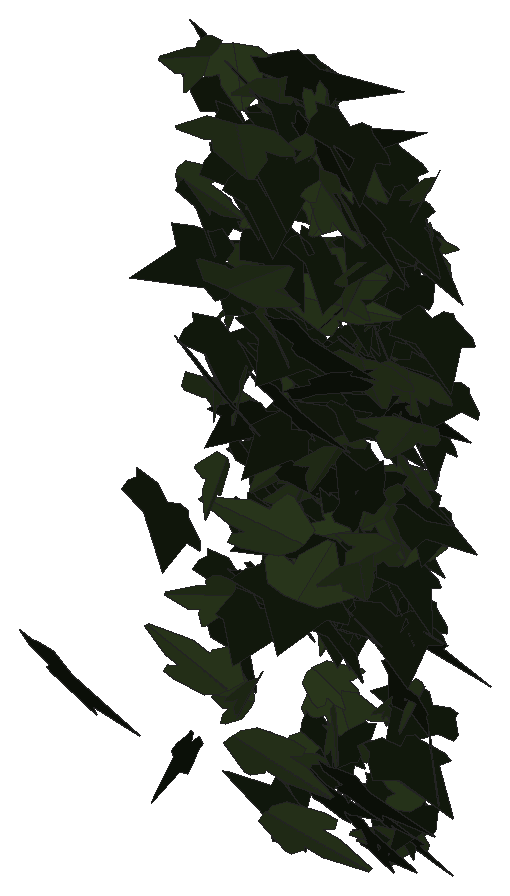
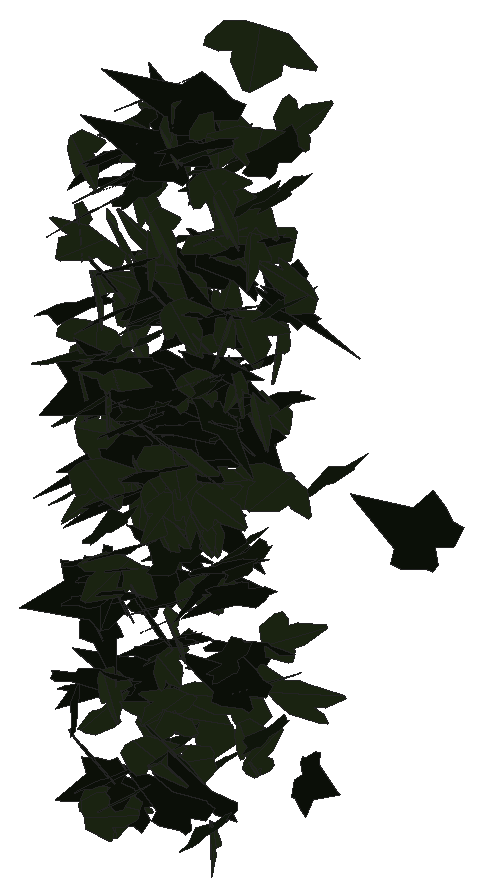
# SketchUp Ruby script. Lengths in millimetres.
U = 1.mm
M = Sketchup.active_model
def pt(a) = Geom::Point3d.new(a.map { |v| v * U })
def face(e, loops, mat)
  f = e.add_face(loops[0].map { |a| pt(a) })
  loops[1..].each { |l| e.add_face(l.map { |a| pt(a) }).erase! }
  f.material = f.back_material = mat if mat
  f
end
# faces: each face lists its corners as indices into pts; further lists are holes
def faces(e, pts, list, mat = nil) = list.each { |f| face(e, (f[0].is_a?(Array) ? f : [f]).map { |l| l.map { |i| pts[i] } }, mat) }
# xy, xz, yz: faces in a plane at the given z, y or x. An outline is a flat list of corners, or four numbers for a rectangle; further outlines are holes
def ring(l) = l.size == 4 ? [[l[0], l[1]], [l[2], l[1]], [l[2], l[3]], [l[0], l[3]]] : l.each_slice(2).to_a
def flat(e, list, mat, &to3) = list.each { |f| face(e, (f[0].is_a?(Array) ? f : [f]).map { |l| ring(l).map { |u, v| to3.(u, v) } }, mat) }
def xy(e, z, list, mat = nil) = flat(e, list, mat) { |x, y| [x, y, z] }
def xz(e, y, list, mat = nil) = flat(e, list, mat) { |x, z| [x, y, z] }
def yz(e, x, list, mat = nil) = flat(e, list, mat) { |y, z| [x, y, z] }
def lines(e, pts, list) = list.each { |a, b| e.add_line(pt(pts[a]), pt(pts[b])) }
# prism: a flat outline (further loops are holes) pulled along v
def prism(e, loops, v, mat = nil)
  f = face(e, loops, mat); d = Geom::Vector3d.new(v.map { |x| x * U })
  f.pushpull(f.normal.samedirection?(d) ? d.length : -d.length)
end
def box(e, o, s, mat = nil) = prism(e, [[o, [o[0] + s[0], o[1], o[2]], [o[0] + s[0], o[1] + s[1], o[2]], [o[0], o[1] + s[1], o[2]]]], [0, 0, s[2]], mat)
def at(x, y, z, deg = 0) = Geom::Transformation.translation(pt([x, y, z])) * Geom::Transformation.rotation(ORIGIN, Z_AXIS, deg.degrees)
def axes(o, x, y, z) = Geom::Transformation.new([*x, 0, *y, 0, *z, 0, *pt(o).to_a, 1])
def part(name) = M.definitions.add(name)
# library, detail: a bought-in or finely detailed component or shape, given as its bounding box
def library(name, o, s) = part(name).tap { |d| box(d.entities, o, s) }
def detail(e, o, s) = box(e.add_group.entities, o, s)
def put(e, d, t, mat = nil) = e.add_instance(d, t).tap { |i| i.material = mat if mat }
def group(e, t, mat = nil) = e.add_group.tap { |g| g.transformation = t; g.material = mat if mat }.entities
root = M.entities
M.materials.add("efeu1").color = [18, 25, 13]
M.materials.add("efeu2").color = [43, 57, 29]
c1 = part("ivyleaf_9")
p = [[39.1,54.8,31.7],[34.5,51.8,30.2],[-5.3,25.2,17.3],[-17.9,28.3,20.9],[-21.6,21.7,17],[-20.2,4.3,5.3],
  [-22.9,-0.3,2.5],[-17.1,-4,-0.6],[-2,-2.1,-1.2],[-0.7,-15.4,-10.1],[16.6,-22.3,-16.7],[21.1,-15.1,-12.5],
  [32.7,-10.7,-11],[46.1,-1.8,-6.6],[30.8,11.2,3.8]]
faces(c1.entities,p,[[0,1,2,3,4,5,6,7,8,9,10,11,12,13,14]],"efeu1")
c2 = part("ivyleaf_10")
p = [[0,12.8,-0.8],[-1.5,51.3,-10.9],[-4.9,51,-11.6],[-13.6,26.5,-7.3],[-13.2,15.9,-4.6],[-21.1,19.3,-7.2],
  [-29.5,16.3,-8.3],[-29.2,8.3,-6.2],[-19.7,-9.8,0.5],[-7.6,-13,4],[1,-12.2,5.8],[-0.4,51.1,-11.1],
  [-1.5,51.1,-10.9],[1,-12.4,5.9],[16.9,-12.4,3.5],[35.1,9.1,-5.1],[35,12.9,-6.1],[20.5,16.4,-4.9],
  [15.8,15,-3.8],[15.3,27.6,-7.1],[12.8,31.3,-7.8]]
faces(c2.entities,p,[[0,1,2,3,4,5,6,7,8,9,10],[11,12,0,13,14,15,16,17,18,19,20]],"efeu2")
put(root,c1,axes([2602.7,851.9,2372.3],[-0.21936,-0.87871,0.39416],[0.01495,-0.39782,-0.88456],[1.83284,-0.10192,0.05439]))
put(root,c1,axes([2606,888.9,1878.8],[-0.45994,-0.83129,0.24224],[0.0835,-0.26293,-0.85853],[1.64581,-0.21897,0.11125]))
put(root,c1,axes([2597.8,883.8,1811],[0.40132,-0.8507,0.15451],[0.01269,-0.15743,-0.8759],[1.64549,0.20869,-0.03093]))
put(root,c2,axes([2606.7,848.6,2133.5],[-1.77967,0.18399,-0.36635],[0.68472,-0.06912,-0.95302],[-0.37405,-1.00191,-0.00152]))
put(root,c2,axes([2620.8,872.2,2243.8],[0.1641,-0.95502,-0.15053],[0.02834,0.15242,-0.95849],[1.83982,0.08284,0.02819]))
put(root,c1,axes([2618.1,790.3,1709],[-0.44208,0.13684,-0.98546],[1.08797,-0.80989,-0.24721],[-1.54976,-0.60759,0.10757]))
put(root,c2,axes([2629.9,801.5,2581.4],[-0.29414,-0.27137,-1.10559],[-0.80082,-1.0231,0.30995],[-2.01318,0.44662,0.03824]))
put(root,c2,axes([2587.1,834.3,2392.7],[-0.07253,0.03539,-1.04948],[1.52236,-0.6794,-0.05196],[-1.29477,-0.8008,-0.0023]))
put(root,c2,axes([2650.2,790.4,1807.9],[1.21959,0.24218,0.89079],[-1.66786,-0.18121,0.67969],[0.55217,-1.08227,0.08553]))
put(root,c2,axes([2641.4,816.1,1895.3],[-0.17895,-0.14003,-1.00925],[-1.12514,-0.818,0.16857],[-1.57943,0.59859,-0.00574]))
put(root,c1,axes([2602.5,840.2,2524.3],[0.83467,-0.89447,-0.20918],[-0.04957,0.2196,-0.99361],[1.74759,0.43344,0.07172]))
put(root,c1,axes([2662.7,790.7,2338.8],[-1.96485,0.28691,0.1811],[-0.33956,0.0343,-1.07142],[-0.54924,-1.04759,0.01452]))
put(root,c1,axes([2615.8,893,2042],[0.65257,-0.84782,0.1484],[0.10051,-0.13872,-0.91452],[1.63502,0.34691,-0.00301]))
put(root,c2,axes([2641.4,857.5,2446],[0.06645,-0.87731,-0.49535],[0.1631,0.49643,-0.87319],[1.91051,-0.01187,0.09177]))
put(root,c1,axes([2613.3,848.2,2566.1],[0.38578,-0.74441,0.64559],[0.59711,-0.57604,-0.76273],[1.77773,0.35503,0.11609]))
put(root,c2,axes([2642.1,853.7,1748],[-0.18778,0.52923,0.88057],[0.34196,-0.8621,0.53826],[1.92516,0.20476,-0.00972]))
put(root,c2,axes([2649.5,882.2,2285.5],[0.87392,-0.77091,-0.40072],[-0.12709,0.42059,-0.88565],[1.64868,0.44106,0.14414]))
put(root,c2,axes([2645.8,875.2,2272.1],[-0.96305,0.80714,0.03517],[-0.01761,0.03571,-0.95257],[-1.5375,-0.50598,-0.01112]))
put(root,c1,axes([2653.1,906.9,2031.1],[-0.85704,-0.76995,0.24056],[-0.14302,-0.23427,-0.89048],[1.52855,-0.45362,0.05156]))
put(root,c1,axes([2646.3,825.7,2223.9],[-0.62993,-0.91874,-0.13351],[0.05549,0.13138,-0.9764],[1.76605,-0.33184,-0.01694]))
put(root,c2,axes([2659.9,848.3,1776],[0.00096,-0.95236,0.04986],[0.00034,-0.04986,-0.95236],[1.815,0.00052,0.00015]))
put(root,c2,axes([2667.4,845.8,2326.4],[-1.12713,-0.8143,0.204],[-0.15951,-0.19105,-1.00594],[1.58969,-0.59653,0.0437]))
put(root,c1,axes([2624.7,891.2,1862.4],[0.54599,-0.24385,0.81417],[1.25459,-0.47854,-0.37561],[1.02098,0.71844,0.02616]))
put(root,c1,axes([2646.8,713.2,2059],[-0.25549,-1.02864,0.62561],[-0.07671,-0.62529,-1.03677],[2.29006,-0.13571,0.03507]))
put(root,c1,axes([2641.6,871.1,1986.9],[0.34993,-0.51268,-0.7806],[0.08361,0.79945,-0.51472],[1.77544,0.0634,0.17809]))
put(root,c2,axes([2659,879.3,2336.6],[0.33743,-0.68183,-0.69468],[0.3058,0.71692,-0.66265],[1.82712,0.00593,0.2392]))
put(root,c1,axes([2680.8,894.3,2292.9],[-1.79147,-0.1632,0.03486],[-0.07173,0.01332,-0.95514],[0.30941,-0.94185,-0.01955]))
put(root,c2,axes([2652.5,829.2,2576.8],[1.51932,0.76395,0.04593],[0.06434,0.03111,-1.10495],[-1.45516,0.79901,-0.0009]))
put(root,c1,axes([2619,549,1914.7],[0.94474,-0.72214,0.98745],[1.06901,-0.81214,-0.8763],[2.06833,0.7496,0.00188]))
put(root,c1,axes([2683.1,877,2215.3],[-0.61302,0.88597,-0.01251],[0.01307,-0.01081,-0.9427],[-1.6863,-0.32216,-0.00276]))
put(root,c1,axes([2655.4,843.9,2435.6],[-0.35308,-1.00084,-0.11203],[0.0424,0.10981,-1.01789],[1.91623,-0.18684,0.00188]))
put(root,c1,axes([2650.6,852.8,2279],[0.34682,-0.92077,-0.42788],[-0.10101,0.42548,-0.93822],[1.92974,0.18776,0.02779]))
put(root,c1,axes([2648.3,883.3,1894.6],[0.94182,-0.7498,0.06909],[0.0776,-0.05587,-0.89837],[1.43095,0.49653,0.00325]))
put(root,c1,axes([2656.4,839,2487.8],[0.17531,-0.969,0.27289],[0.08006,-0.27008,-0.97324],[1.91426,0.10004,0.01571]))
put(root,c2,axes([2678.5,869.3,2488],[0.44902,-0.97411,0.15207],[0.06468,-0.14824,-1.00227],[1.87527,0.23836,-0.00184]))
put(root,c1,axes([2680.4,834.6,1882.8],[-1.20928,-0.64803,-0.07539],[0.10298,0.05252,-0.90756],[1.23736,-0.63769,0.00186]))
put(root,c2,axes([2682.5,880.9,1649.4],[0.44059,-0.74472,-0.50283],[0.01518,0.52094,-0.76786],[1.71011,0.18724,0.13637]))
put(root,c2,axes([2670.6,816.1,2182],[0.70923,-0.63127,0.66398],[0.68561,-0.55811,-0.73279],[1.60321,0.51793,0.01964]))
put(root,c2,axes([2681.4,822.4,2472.4],[-1.96824,0.26821,-0.24851],[0.45899,-0.06,-1.06839],[-0.52306,-1.06192,-0.0024]))
put(root,c1,axes([2673.2,906.2,1661.4],[0.07009,-0.86836,0.3748],[-0.0412,-0.37576,-0.86845],[1.79955,0.02522,-0.03448]))
put(root,c1,axes([2708.5,811.3,2153.3],[0.26368,0.62848,-0.82882],[-0.47805,-0.79118,-0.64192],[-1.92103,0.28315,0.04598]))
put(root,c2,axes([2698.6,865.8,2512.7],[-0.7251,-0.88498,0.32547],[-0.01409,-0.34822,-0.95549],[1.79453,-0.36032,0.12401]))
put(root,c1,axes([2676.6,825.7,2014.3],[0.85335,-0.85765,-0.3751],[-0.31251,0.3374,-0.96773],[1.75394,0.47739,0.01007]))
put(root,c1,axes([2690.4,868.7,1986.1],[0.63778,-0.48439,-0.83189],[-0.76032,0.73144,-0.58683],[1.66688,0.51897,0.05062]))
put(root,c1,axes([2680.7,874.8,2256.2],[0.32728,-0.92549,0.15648],[0.03045,-0.15617,-0.94125],[1.78614,0.17224,-0.01263]))
put(root,c2,axes([2711.2,854.1,2075.8],[-0.36736,-0.69607,0.67241],[-0.26741,-0.65823,-0.72173],[1.82242,-0.2369,0.02964]))
put(root,c1,axes([2675.1,845.6,2196.2],[0.85438,-0.86585,0.1528],[0.15317,-0.13038,-0.97524],[1.66632,0.45593,0.0113]))
put(root,c2,axes([2711.2,838.5,2421.2],[1.3122,0.52505,-0.56863],[-0.85221,-0.35053,-0.86661],[-1.20145,0.82209,-0.00634]))
put(root,c1,axes([2709.9,900.4,2196.5],[-1.12055,-0.74701,0.11521],[-0.07552,-0.11529,-0.95031],[1.43654,-0.58876,0.03991]))
put(root,c1,axes([2705.1,874.1,2249],[-0.63639,-0.80058,0.39494],[-0.09437,-0.40443,-0.8618],[1.69635,-0.32284,0.10022]))
put(root,c1,axes([2700.3,827.6,2427.8],[-0.36829,-0.99153,0.12935],[0.03974,-0.13573,-1.00919],[1.90266,-0.18909,0.04612]))
put(root,c2,axes([2712.3,714.3,2237.3],[0.75529,-0.74713,-0.71349],[0.11803,0.78017,-0.78246],[1.96263,0.2406,0.32163]))
put(root,c2,axes([2716.1,824.3,2567.7],[-1.07398,-0.83663,-0.16183],[0.17456,0.13334,-1.00915],[1.61237,-0.5717,0.00146]))
put(root,c2,axes([2721.8,863.3,1959.1],[-0.8275,-0.6079,0.53089],[-0.03967,-0.59436,-0.69766],[1.53554,-0.34295,0.26807]))
put(root,c2,axes([2722.7,847.3,2043.2],[-0.2692,-0.89225,0.21418],[0.06119,-0.2214,-0.90107],[1.74529,-0.12986,0.06463]))
put(root,c2,axes([2720.2,863,2044.2],[-0.08012,-0.86376,0.32622],[0.16338,-0.32881,-0.85953],[1.74963,-0.00885,0.0952]))
put(root,c1,axes([2696.9,836.8,2511.4],[0.7449,-0.9047,-0.11968],[0.00858,0.13214,-0.98413],[1.7368,0.38737,0.05619]))
put(root,c2,axes([2727.2,891.9,2338.7],[-0.41673,-0.903,0.26053],[-0.09602,-0.25583,-0.9291],[1.7861,-0.22444,0.01084]))
put(root,c2,axes([2721.9,838.3,2309.6],[-1.54178,-0.6012,-0.27155],[0.40626,0.16801,-1.00879],[1.18797,-0.83771,-0.00744]))
put(root,c1,axes([2715.8,865.9,1675.8],[-1.2914,0.37308,0.5768],[0.89547,-0.33831,0.77232],[0.95258,0.82381,0.05594]))
put(root,c1,axes([2706.7,866.5,2327.1],[-0.17094,-0.77049,-0.6316],[0.25426,0.61912,-0.77427],[1.879,-0.15387,0.04731]))
put(root,c2,axes([2718.6,717.5,2126.7],[-0.02832,-0.76302,0.78628],[0.65781,-0.74947,-0.72075],[1.97875,0.23823,0.25086]))
put(root,c1,axes([2706,844.4,2301.6],[-0.46181,0.39278,0.92671],[0.71503,-0.84901,0.45822],[1.77714,0.44367,0.05645]))
put(root,c1,axes([2708.6,871.7,2564.9],[0.00716,-0.93278,-0.39109],[0.25402,0.38813,-0.92444],[1.90816,-0.04817,0.12453]))
put(root,c2,axes([2737.8,858.7,2074.8],[-0.29774,-1.00667,-0.02735],[0.01379,0.02656,-1.01875],[1.91656,-0.15658,0.00308]))
put(root,c2,axes([2735.3,893.7,1920.4],[0.64883,-0.83939,-0.00188],[0.00844,0.00383,-0.90596],[1.5975,0.3409,0.00555]))
put(root,c1,axes([2714.9,679.2,2280],[1.91372,-0.57363,-0.42942],[-0.70249,0.21958,-1.15762],[1.1689,1.07111,0.00734]))
put(root,c1,axes([2725.3,843.5,2533.8],[-0.56061,-0.83063,0.51097],[0.12107,-0.549,-0.85578],[1.85206,-0.21554,0.21061]))
put(root,c1,axes([2728.4,908.2,1932.4],[-0.35387,-0.84422,0.35375],[-0.10126,-0.3504,-0.86418],[1.73913,-0.19218,0.02166]))
put(root,c2,axes([2740.7,850.1,2219.7],[-0.52454,-0.83124,0.55958],[0.14083,-0.59566,-0.84839],[1.90188,-0.18515,0.21715]))
put(root,c1,axes([2748.8,801.8,2149.6],[-1.73822,0.19062,-0.36483],[0.67867,-0.07713,-0.93299],[-0.39134,-0.98046,0.00247]))
put(root,c2,axes([2765.7,769,2038.9],[0.76,0.52464,1.03967],[-1.26191,-0.80112,0.65893],[1.82204,-0.77368,0.0227]))
put(root,c2,axes([2738.4,902,1867.4],[-0.10446,-0.73977,0.53334],[0.31137,-0.53362,-0.72333],[1.70753,0.05205,0.16453]))
put(root,c1,axes([2717.8,813.2,2381.7],[-0.80055,-0.24656,-0.92627],[1.80363,0.04474,-0.44227],[0.27361,-1.01632,0.20525]))
put(root,c1,axes([2718.5,902.4,2012.7],[0.24235,-0.75514,0.53029],[0.43144,-0.49331,-0.75691],[1.70234,0.23253,0.11634]))
put(root,c1,axes([2745.7,829.3,2496.7],[-1.04861,-0.62266,0.728],[-0.35671,-0.75352,-0.78634],[1.78795,-0.51551,0.27008]))
put(root,c1,axes([2768.2,888.9,2160.2],[-1.62005,0.40612,0.03095],[-0.13797,-0.08051,-0.93741],[-0.7628,-0.84797,0.10382]))
put(root,c2,axes([2754.6,867.8,2125],[-1.59628,-0.38878,0.14588],[-0.2393,-0.07558,-0.92433],[0.7532,-0.84797,0.01551]))
put(root,c1,axes([2738.2,838.3,2476.9],[-0.36713,-0.03737,1.02446],[-0.1822,-1.03723,-0.05586],[1.94253,-0.10435,0.18838]))
put(root,c2,axes([2727.4,845.5,1715.9],[-0.15918,-0.11898,-0.91944],[1.17068,0.68359,-0.14442],[1.32016,-0.62053,0.0172]))
put(root,c1,axes([2773,842,2298.9],[-1.46345,0.3736,-0.61075],[-1.04256,0.27009,0.85489],[0.87737,0.94411,-0.00288]))
put(root,c1,axes([2775.5,805.3,2025.9],[0.43176,0.16561,-1.03235],[-1.4954,-0.66991,-0.28013],[-1.31279,0.81757,-0.02043]))
put(root,c1,axes([2762.3,793.9,1666.3],[-0.07811,-1.04362,-0.04959],[0.01653,-0.04997,1.04437],[-1.98839,0.04058,0.01063]))
put(root,c2,axes([2752.7,773.2,2270.5],[-1.58975,0.70766,0.13036],[0.17014,-0.09612,1.09466],[1.35887,0.83993,0.01545]))
put(root,c1,axes([2727.1,855.1,2015.3],[1.01737,-0.72192,-0.21192],[-0.05691,0.23937,-0.89086],[1.4308,0.52284,0.11525]))
put(root,c1,axes([2741.2,886.8,1891.1],[-0.46485,-0.86165,-0.14163],[0.054,0.13916,-0.89554],[1.66102,-0.24566,-0.01052]))
put(root,c1,axes([2736.1,883.2,2006.5],[0.4226,-0.8651,-0.19712],[-0.11894,0.18744,-0.89304],[1.68446,0.23027,-0.0136]))
put(root,c2,axes([2733.4,736.2,2355],[-1.6719,-0.55676,0.57833],[1.05221,0.20201,1.03426],[-1.10777,1.03216,0.10954]))
put(root,c1,axes([2754.6,820.9,1945.9],[-1.44548,-0.77644,-0.16308],[0.21474,0.11776,-1.08614],[1.49462,-0.76783,-0.00167]))
put(root,c2,axes([2759.5,879.9,2037.5],[1.33451,-0.53462,-0.30281],[-0.31051,0.28097,-0.87385],[1.12739,0.71022,0.11776]))
put(root,c2,axes([2749.6,873.3,2063.1],[-0.61232,-0.71471,-0.68752],[0.67291,0.59264,-0.78152],[1.7634,-0.47432,0.05949]))
put(root,c1,axes([2792.4,838.5,2171],[-1.75389,-0.20828,-0.4318],[-0.8026,-0.09281,0.94479],[-0.43395,1.01345,-0.00222]))
put(root,c1,axes([2749.1,890.3,1937.7],[-0.48016,-0.85266,0.19023],[0.07408,-0.20878,-0.88418],[1.66103,-0.23717,0.09442]))
put(root,c1,axes([2726.1,875,1655.5],[0.39822,-0.3432,0.85894],[1.08974,-0.64357,-0.39663],[1.38256,0.60612,0.06522]))
put(root,c2,axes([2745.4,869.7,1803.9],[0.53531,0.73337,0.51824],[0.38364,0.47764,-0.78532],[-1.66545,0.34575,-0.01433]))
put(root,c2,axes([2781.6,885.6,1727.4],[-0.88868,-0.4314,0.62761],[-0.87254,-0.42862,-0.63572],[1.15739,-0.65438,0.00264]))
put(root,c1,axes([2753.1,900.8,1886],[-0.47819,-0.88041,-0.04633],[0.02189,0.0449,-0.91556],[1.67778,-0.25152,-0.00126]))
put(root,c1,axes([2743,880.8,1879.2],[0.4374,-0.87455,0.01617],[0.00837,-0.01557,-0.90425],[1.66471,0.22987,0.0003]))
put(root,c2,axes([2770.3,875.4,2077],[-0.39273,-0.82514,0.38375],[-0.14479,-0.37647,-0.85041],[1.72587,-0.21935,0.01598]))
put(root,c1,axes([2791,840.8,2207.7],[-0.18523,0.05044,1.04927],[-1.90244,-0.32843,-0.07693],[0.61469,-1.00129,0.07809]))
put(root,c1,axes([2729.6,807.7,2176],[0.67307,-0.53428,0.84873],[0.97864,-0.67605,-0.63984],[1.63872,0.62318,0.03352]))
put(root,c1,axes([2769.2,790,2279.6],[-1.08532,-0.75318,0.37312],[-0.16461,-0.39592,-0.93138],[1.59121,-0.55468,0.15814]))
put(root,c2,axes([2772.3,870.8,2432.7],[0.24487,-0.99177,0.13567],[-0.00161,-0.1369,-0.99991],[1.90512,0.12736,-0.01828]))
put(root,c1,axes([2751.5,875.6,1734.7],[0.1275,-0.97796,0.37851],[0.02741,-0.37838,-0.98019],[1.99561,0.06768,-0.01072]))
put(root,c2,axes([2734.7,761,1761.1],[-1.14756,0.10314,-1.02967],[1.92973,-0.17936,-0.61172],[-0.39372,-1.17967,0.00298]))
put(root,c1,axes([2729.2,827.6,2574.8],[0.55015,-0.0248,1.07842],[2.02917,-0.16304,-0.28954],[0.31188,1.10452,-0.01853]))
put(root,c1,axes([2764.4,775.7,2516.5],[-0.61307,-1.05615,-0.06929],[0.03486,0.06685,-1.10418],[2.01409,-0.32264,-0.00198]))
put(root,c1,axes([2803.4,869.4,1914],[-0.88816,0.23696,-0.90256],[-1.59524,0.33707,0.52188],[0.78054,0.95852,0.0396]))
put(root,c2,axes([2769.6,857.2,2548.2],[0.63927,-0.83895,0.45568],[0.36289,-0.41437,-0.90346],[1.78041,0.38569,0.02053]))
put(root,c1,axes([2801.9,853.3,1746.5],[-1.02056,0.78745,0.25666],[-0.31157,0.19895,-0.95242],[-1.54517,-0.56021,0.02253]))
put(root,c1,axes([2768.9,878.4,2104.2],[-0.63357,-0.87532,-0.0189],[0.01434,0.01735,-0.93649],[1.66624,-0.33298,0.00088]))
put(root,c2,axes([2784.4,854.2,2011.3],[-0.26579,0.04739,0.94196],[-0.21679,-0.94611,0.03071],[1.78187,-0.10804,0.14424]))
put(root,c2,axes([2781.4,674.3,2594.8],[-2.21566,-0.48141,-0.08027],[0.13984,0.03237,-1.25978],[0.91829,-1.16649,-0.00183]))
put(root,c2,axes([2761.3,875.5,1777],[1.64432,0.29336,0.24652],[0.43303,0.09651,-0.91225],[-0.58681,0.89326,0.0176]))
put(root,c1,axes([2800.4,840.6,1987.9],[-2.00035,-0.0233,-0.03402],[0.06484,-0.00168,-1.0513],[0.04423,-1.0516,0.00243]))
put(root,c2,axes([2784,812.6,2553.7],[0.01539,0.67421,-0.8208],[0.07808,0.82001,0.67397],[2.02008,-0.03683,-0.01979]))
put(root,c1,axes([2740.3,809.6,2096],[0.69289,-0.12693,0.98829],[1.72891,-0.39001,-0.38473],[0.77912,0.97834,-0.02516]))
put(root,c1,axes([2777.8,857.8,2074.5],[-0.51641,-0.6118,0.70407],[-0.06252,-0.72653,-0.64398],[1.7741,-0.20369,0.18225]))
put(root,c2,axes([2787.7,807.3,2531.4],[-0.05433,-0.9126,0.48072],[0.18133,-0.48118,-0.90782],[1.95471,0.01927,0.09758]))
put(root,c1,axes([2770.6,864.8,2316.1],[0.29556,-0.91969,-0.25782],[0.03895,0.26435,-0.93065],[1.81741,0.1439,0.06187]))
put(root,c1,axes([2774.1,877.7,2308.6],[0.02201,-0.96239,0.23269],[0.13842,-0.23125,-0.96005],[1.8793,0.0283,0.06799]))
put(root,c2,axes([2777.5,844.4,1767.6],[0.27702,-0.23843,1.00634],[1.2112,-0.78042,-0.27695],[1.55151,0.65181,0.03652]))
put(root,c1,axes([2769.8,841.7,2157.7],[-0.52551,-0.13522,1.02177],[1.85545,-0.37751,0.21349],[0.63652,0.98881,0.22124]))
put(root,c1,axes([2776.3,882.9,2191.5],[0.36862,-0.85237,0.3665],[0.47779,-0.31229,-0.85897],[1.69997,0.2726,0.16194]))
put(root,c1,axes([2765.9,838.3,2504.6],[0.32372,-0.12784,1.09766],[2.0911,0.13846,-0.15413],[-0.22517,1.1021,0.14669]))
put(root,c1,axes([2794.1,821.3,2377.9],[-0.52643,-0.89027,0.39213],[0.0322,-0.41202,-0.92348],[1.85117,-0.24601,0.12758]))
put(root,c1,axes([2801.3,823.1,2306.2],[0.44242,0.60482,0.83454],[0.621,0.76832,-0.64771],[-1.86066,0.40024,-0.01774]))
put(root,c2,axes([2809.3,800.5,2141.4],[-0.29401,-0.97061,0.22397],[-0.01965,-0.22508,-0.98252],[1.89571,-0.15287,0.02455]))
put(root,c2,axes([2805.6,842.7,2384.2],[0.91074,-0.71819,-0.51175],[0.04306,0.59205,-0.80972],[1.67781,0.37465,0.29857]))
put(root,c1,axes([2790.9,896.6,2273.4],[-0.10311,-0.91368,0.2806],[0.12938,-0.28402,-0.91169],[1.81446,-0.03167,0.08095]))
put(root,c2,axes([2808.8,870.8,2273.5],[0.4484,-0.92098,0.12448],[0.03949,-0.12317,-0.95058],[1.7683,0.23629,-0.01034]))
put(root,c1,axes([2791.7,893.7,2168.9],[0.05225,-0.93901,-0.13122],[0.02972,0.1317,-0.93921],[1.80424,0.02502,0.01927]))
put(root,c2,axes([2793.2,771.3,1980.1],[1.37139,0.6946,-0.56781],[0.78273,0.39151,1.00084],[1.51749,-0.82967,-0.00309]))
put(root,c2,axes([2801.3,890.7,2268.7],[-0.51679,0.903,-0.16027],[0.14888,-0.14373,-0.94237],[-1.7391,-0.28064,-0.03305]))
put(root,c1,axes([2775.7,878.9,2202.9],[0.05361,-0.10496,0.97462],[1.61603,-0.48457,-0.07673],[0.93218,0.84609,0.07696]))
put(root,c1,axes([2786.8,854,1912.5],[0.13053,-0.50346,0.80513],[0.63504,-0.74297,-0.49302],[1.69199,0.31769,0.12293]))
put(root,c1,axes([2811.4,896.8,2244.1],[-0.96556,-0.8205,-0.11291],[0.08736,0.10435,-0.96455],[1.57386,-0.50916,-0.01573]))
put(root,c2,axes([2777.4,812.5,2323.2],[0.00341,-0.25574,-1.11141],[2.06286,0.34606,-0.07788],[0.67509,-1.05616,0.24359]))
put(root,c1,axes([2794,800.1,2516.3],[-0.28142,-0.05844,1.06242],[0.67955,-1.01315,-0.00604],[1.90762,0.35229,0.15888]))
put(root,c1,axes([2810.7,902.9,1654.8],[-0.3392,-0.72956,0.40766],[-0.11179,-0.40486,-0.75023],[1.58663,-0.1845,0.03429]))
put(root,c1,axes([2818.8,903.6,1988.7],[-0.67283,-0.77644,0.33534],[-0.13637,-0.33466,-0.85039],[1.60387,-0.35418,0.06837]))
put(root,c1,axes([2810,867.6,2060.3],[-0.11764,-0.96213,-0.06134],[0.00371,0.06134,-0.96411],[1.83484,-0.06181,-0.00198]))
put(root,c1,axes([2821.6,878.7,2362.9],[-0.73622,-0.82016,0.34818],[-0.11601,-0.35433,-0.90237],[1.69179,-0.38121,0.08964]))
put(root,c2,axes([2846.4,897.8,1622.7],[-0.33885,0.12447,-0.83945],[-1.14111,-0.62545,0.03443],[-1.14299,0.58752,0.21449]))
put(root,c2,axes([2818,883.9,1959.8],[-1.30992,-0.54516,-0.57548],[0.8722,0.3482,-0.87796],[1.23099,-0.82683,0.0097]))
put(root,c2,axes([2826.1,885.9,2218.8],[1.77596,0.17375,-0.09025],[-0.16327,-0.03221,-0.94905],[-0.33495,0.93695,-0.01589]))
put(root,c2,axes([2834.5,889.2,1804.5],[-0.03961,-0.91207,-0.09024],[-0.01505,0.09044,-0.91225],[1.74425,-0.01993,-0.00992]))
put(root,c1,axes([2807.3,853.4,2181.4],[0.63584,-0.7499,-0.56726],[0.07704,0.61292,-0.78641],[1.78789,0.24028,0.23562]))
put(root,c2,axes([2827.2,811.7,2505.7],[1.97361,-0.24997,-0.04703],[-0.08557,0.01419,-1.06669],[0.47647,1.03796,0.00325]))
put(root,c2,axes([2835.3,792.8,2483.7],[1.21774,0.6897,-0.53895],[-0.68739,-0.40007,-0.94076],[-1.51743,0.73471,-0.00635]))
put(root,c1,axes([2814.8,882.7,2311.1],[0.51416,-0.85523,-0.40836],[-0.02769,0.42083,-0.89098],[1.80348,0.25028,0.10274]))
put(root,c2,axes([2800,818.9,2351],[1.04975,-0.3833,-0.89635],[1.45673,-0.46754,0.67093],[-1.14905,-0.94291,0.03169]))
put(root,c1,axes([2822.6,845.4,2444.9],[-0.30617,-0.71802,0.7517],[0.06032,-0.76368,-0.72268],[1.9775,-0.08787,0.13843]))
put(root,c1,axes([2851.6,855,1910.3],[-0.04009,0.40421,0.86753],[-0.16043,0.86358,-0.40442],[-1.81442,-0.08529,0.01659]))
put(root,c1,axes([2797.3,757.8,2295.3],[0.4979,-0.37446,0.95509],[1.29356,-0.67502,-0.45083],[1.46245,0.72456,0.0736]))
put(root,c1,axes([2832.4,874.3,2467.1],[-0.71921,-0.8089,0.46344],[-0.1388,-0.47288,-0.88486],[1.76883,-0.36601,0.119]))
put(root,c2,axes([2844.9,874.1,1636.9],[-1.26719,-0.57985,0.08363],[-0.11318,-0.05906,-0.8829],[1.10923,-0.66845,0.00546]))
put(root,c2,axes([2799.4,740.6,1696.8],[-0.92308,0.1138,-1.0983],[2.05347,-0.20608,-0.49782],[-0.44658,-1.18281,-0.01893]))
put(root,c2,axes([2849.6,898.3,2085.4],[-0.89382,-0.72041,0.42452],[-0.26251,-0.41349,-0.85427],[1.56964,-0.47938,0.09887]))
put(root,c1,axes([2805.5,861,1633.9],[1.00429,-0.13411,-0.73594],[1.40361,-0.0575,0.53928],[-0.23834,-0.90374,0.07489]))
put(root,c1,axes([2829.3,898,2012.2],[-0.24169,-0.71118,0.61671],[-0.03452,-0.62033,-0.71909],[1.7912,-0.10791,0.06936]))
put(root,c1,axes([2843,885.2,1943.8],[-0.96369,-0.73157,0.28551],[-0.20379,-0.27222,-0.88743],[1.48065,-0.51362,0.06369]))
put(root,c1,axes([2827.9,894.3,1678.6],[-0.08295,-0.93003,-0.03017],[0.0068,0.03004,-0.93105],[1.77095,-0.04368,0.00216]))
put(root,c1,axes([2847.8,863.3,1948.1],[1.03587,-0.26203,-0.88304],[-1.5158,0.38135,-0.60406],[0.88059,0.96466,-0.00106]))
put(root,c1,axes([2819.5,835.2,2091.4],[0.1147,0.00922,-1.05526],[0.60433,1.00784,0.02694],[1.91538,-0.31854,0.05469]))
put(root,c1,axes([2843.4,901.5,1920.3],[-0.78166,-0.80099,0.01291],[-0.01135,-0.01145,-0.90014],[1.52459,-0.41075,-0.00008]))
put(root,c2,axes([2849.6,868.8,2176.1],[0.45125,-0.77248,-0.49054],[0.01833,0.50882,-0.79661],[1.74147,0.19481,0.13549]))
put(root,c1,axes([2833.1,805.7,2559.4],[-0.19263,-1.0861,0.17831],[0.00486,-0.17929,-1.09064],[2.09473,-0.09946,0.01893]))
put(root,c2,axes([2850.4,854.1,2393.2],[1.08796,-0.87708,0.00525],[-0.00005,-0.00628,-1.04692],[1.66928,0.57164,-0.00345]))
put(root,c1,axes([2832.4,869.5,2043.4],[0.4878,-0.73221,-0.599],[-0.02559,0.61771,-0.76084],[1.80026,0.20718,0.15149]))
put(root,c2,axes([2859.4,880,2328.6],[0.48622,-0.8284,-0.44473],[-0.10871,0.44633,-0.86419],[1.78614,0.25267,0.06846]))
put(root,c2,axes([2857.8,790,2019.9],[-0.76637,-0.98545,-0.34394],[0.24567,0.3188,-1.06455],[1.97121,-0.42286,-0.00104]))
put(root,c1,axes([2841.6,732.7,2270.7],[1.2158,0.73595,0.6306],[0.74712,0.49405,-0.97426],[-1.68643,0.74944,0.02301]))
put(root,c1,axes([2840.1,858.7,2504.7],[0.25418,-0.94746,-0.32727],[0.07679,0.33498,-0.95331],[1.90621,0.11285,0.08204]))
put(root,c1,axes([2839.1,847.1,2468.1],[0.75647,-0.85339,-0.43074],[-0.15679,0.43417,-0.93621],[1.81256,0.39372,0.09878]))
put(root,c1,axes([2838.6,865.2,1655.7],[1.54817,-0.27877,0.04132],[0.07462,-0.01305,-0.8599],[0.53114,0.8144,0.00037]))
put(root,c2,axes([2879.8,807.8,2044.9],[-0.97973,-0.59187,0.52175],[-0.55566,-0.43587,-0.7825],[1.39504,-0.58927,0.05475]))
put(root,c1,axes([2866.2,819.5,2443.8],[-0.99842,-0.89633,0.25874],[-0.23057,-0.22887,-1.03851],[1.76051,-0.5383,0.01072]))
put(root,c1,axes([2874.4,894.5,1802.7],[-1.27185,-0.54794,0.11511],[-0.1448,-0.08871,-0.86395],[1.05571,-0.67228,0.02018]))
put(root,c2,axes([2865.6,783.5,2400.1],[0.08569,-0.94848,0.37058],[0.25856,-0.36203,-0.94311],[1.92071,0.09105,0.11042]))
put(root,c1,axes([2873.3,875.5,2355.2],[-1.52222,0.24945,-0.51189],[0.89619,-0.20653,-0.83641],[-0.60938,-0.92687,0.04861]))
put(root,c2,axes([2829.2,765.8,2493.4],[0.42804,-0.08428,1.21566],[2.02416,-0.5898,-0.23766],[1.13199,1.08652,-0.03472]))
put(root,c1,axes([2892.9,752.7,2123.3],[-0.17033,0.57934,1.11363],[-0.35493,1.09793,-0.58616],[-2.3626,-0.20671,0.00777]))
put(root,c1,axes([2885.2,842.5,1850.9],[0.72156,-0.0199,-0.91772],[-1.72397,0.15265,-0.37752],[0.28286,0.98115,0.04012]))
put(root,c2,axes([2894.8,852.5,2107.2],[-0.52157,0.55462,-0.9475],[-1.05102,0.7744,0.61302],[1.80592,0.61087,0.08313]))
put(root,c2,axes([2870.5,789.4,2278.8],[-1.93805,0.00515,-0.09705],[0.18469,-0.00231,-1.01832],[-0.01017,-1.02292,0.00181]))
put(root,c2,axes([2841.6,836.4,2073.9],[1.03392,-0.33773,0.8446],[1.49977,-0.31665,-0.63348],[0.86472,0.953,0.08883]))
put(root,c1,axes([2849.9,863.8,2181.2],[1.51462,0.38797,0.34315],[0.61574,0.1189,-0.88476],[-0.76979,0.85846,-0.03254]))
put(root,c1,axes([2865,847.3,1931.2],[-0.94042,-0.69278,-0.4438],[0.46639,0.37026,-0.85083],[1.49477,-0.55139,-0.01374]))
put(root,c2,axes([2880.9,809.6,2098.5],[-0.38811,-0.51942,-0.76545],[-0.58139,-0.70205,0.55778],[-1.66179,0.36693,-0.01637]))
put(root,c2,axes([2883,852.8,2240.2],[-1.81576,0.0196,0.0646],[-0.12606,-0.09508,-0.9494],[-0.02481,-0.9515,0.0962]))
put(root,c2,axes([2883.3,855,1714.8],[-0.06666,0.77467,0.6225],[-0.06388,-0.62345,0.77397],[1.8903,0.00625,0.04811]))
put(root,c1,axes([2885.1,870.5,1688.9],[-1.34102,0.24131,-0.4589],[0.79874,-0.18919,-0.74389],[-0.57941,-0.81931,0.03662]))
put(root,c2,axes([2852.5,886.8,2389.3],[1.43493,0.17984,0.59982],[1.05071,0.25216,-0.76955],[-0.56246,0.92987,0.09268]))
put(root,c1,axes([2867.6,896.6,2160.1],[-0.05344,-0.90071,0.3593],[0.0235,-0.35976,-0.90088],[1.84544,-0.0215,0.02187]))
put(root,c1,axes([2873.1,898.6,2051],[-0.35836,-0.87979,0.447],[-0.10578,-0.44489,-0.89904],[1.87515,-0.19323,0.03471]))
put(root,c2,axes([2883.1,852.1,2023.8],[-0.14026,0.28472,1.03336],[-0.31625,1.02025,-0.29295],[-2.01532,-0.17992,-0.02595]))
put(root,c1,axes([2850.5,872.8,1906.4],[1.8783,-0.25548,0.22779],[0.42995,-0.0361,-1.01923],[0.48941,1.01222,0.02114]))
put(root,c2,axes([2901,824.9,2196.1],[-1.31687,-0.60066,0.27656],[-0.37823,-0.19289,-0.91615],[1.20035,-0.71975,0.01473]))
put(root,c2,axes([2887.4,875.6,2406.2],[0.44521,-0.93139,-0.19948],[0.16921,0.22586,-0.95031],[1.8049,0.20857,0.1383]))
put(root,c1,axes([2849,779.3,1742.4],[0.93593,-0.46473,0.78965],[1.18403,-0.48859,-0.67498],[1.28023,0.79163,0.04698]))
put(root,c2,axes([2892.3,867.8,2185.3],[0.6226,-0.84864,-0.28411],[0.004,0.30322,-0.90332],[1.70323,0.3095,0.10597]))
put(root,c1,axes([2873.3,861.3,2070.1],[0.73414,-0.46473,-0.76294],[-0.27868,0.7869,-0.55336],[1.67721,0.33417,0.24201]))
put(root,c1,axes([2872.5,862.1,2416.5],[0.62915,-0.8505,-0.42959],[-0.132,0.43203,-0.90869],[1.80862,0.32738,0.08312]))
put(root,c1,axes([2873.6,847.8,1768],[0.01873,-0.78855,-0.55731],[0.29126,0.55157,-0.77772],[1.81452,-0.08039,0.13059]))
put(root,c1,axes([2876,826.1,2472.5],[0.31965,-0.91073,-0.55695],[-0.14772,0.5519,-0.92587],[2.02636,0.1839,0.02036]))
put(root,c1,axes([2883.1,889.7,2296.5],[-0.28174,-0.95082,-0.18639],[0.0615,0.1836,-0.96227],[1.84302,-0.15148,0.00362]))
put(root,c2,axes([2899.4,861.8,2489.3],[0.04309,-1.00792,0.16981],[0.04114,-0.16934,-1.00802],[1.94488,0.02591,0.01756]))
put(root,c1,axes([2871.1,769.4,2488.4],[0.90343,-0.9316,0.0422],[0.03135,-0.03897,-1.04556],[1.77456,0.47496,-0.00301]))
put(root,c1,axes([2892.5,896.1,2220.2],[-0.85445,-0.79228,0.37654],[0.17341,-0.46282,-0.86518],[1.66046,-0.35936,0.28412]))
put(root,c1,axes([2880.9,890.2,1755.2],[0.07669,-0.11201,-0.9374],[1.51891,-0.49716,0.09371],[-0.95981,-0.79572,0.0734]))
put(root,c1,axes([2883.8,840.8,2011.4],[0.18288,-0.96582,-0.0051],[-0.0009,0.00507,-0.97059],[1.83817,0.09609,0.00003]))
put(root,c2,axes([2901.3,837.6,1852.5],[0.77422,-0.87935,0.13467],[0.09529,-0.12521,-0.96886],[1.6904,0.40981,-0.00706]))
